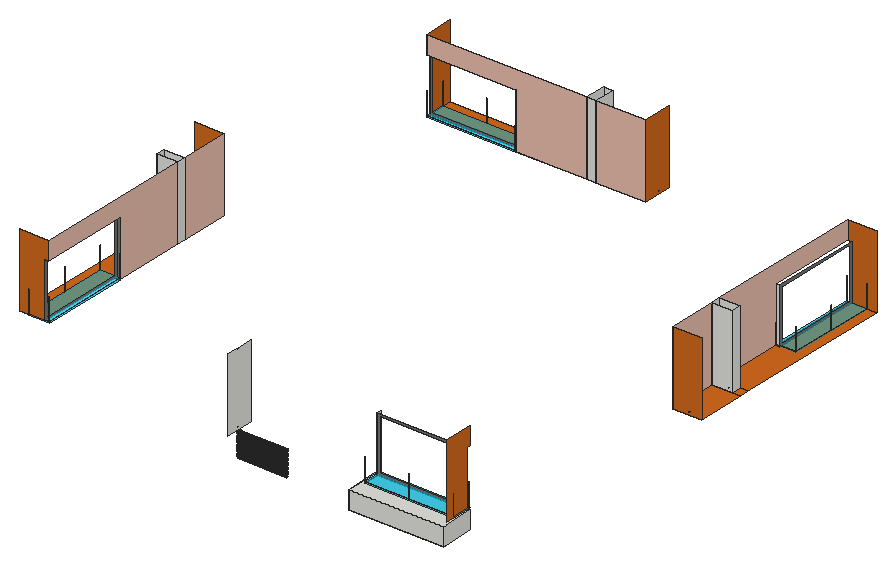
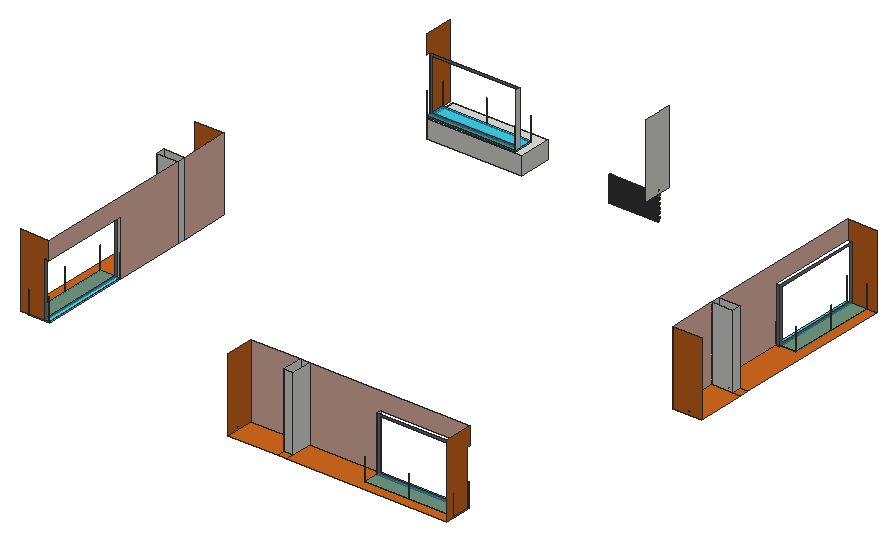
# SketchUp Ruby script. Lengths in inches.
U = 1.inch
M = Sketchup.active_model
def pt(a) = Geom::Point3d.new(a.map { |v| v * U })
def face(e, loops, mat)
  f = e.add_face(loops[0].map { |a| pt(a) })
  loops[1..].each { |l| e.add_face(l.map { |a| pt(a) }).erase! }
  f.material = f.back_material = mat if mat
  f
end
# faces: each face lists its corners as indices into pts; further lists are holes
def faces(e, pts, list, mat = nil) = list.each { |f| face(e, (f[0].is_a?(Array) ? f : [f]).map { |l| l.map { |i| pts[i] } }, mat) }
# xy, xz, yz: faces in a plane at the given z, y or x. An outline is a flat list of corners, or four numbers for a rectangle; further outlines are holes
def ring(l) = l.size == 4 ? [[l[0], l[1]], [l[2], l[1]], [l[2], l[3]], [l[0], l[3]]] : l.each_slice(2).to_a
def flat(e, list, mat, &to3) = list.each { |f| face(e, (f[0].is_a?(Array) ? f : [f]).map { |l| ring(l).map { |u, v| to3.(u, v) } }, mat) }
def xy(e, z, list, mat = nil) = flat(e, list, mat) { |x, y| [x, y, z] }
def xz(e, y, list, mat = nil) = flat(e, list, mat) { |x, z| [x, y, z] }
def yz(e, x, list, mat = nil) = flat(e, list, mat) { |y, z| [x, y, z] }
def lines(e, pts, list) = list.each { |a, b| e.add_line(pt(pts[a]), pt(pts[b])) }
# prism: a flat outline (further loops are holes) pulled along v
def prism(e, loops, v, mat = nil)
  f = face(e, loops, mat); d = Geom::Vector3d.new(v.map { |x| x * U })
  f.pushpull(f.normal.samedirection?(d) ? d.length : -d.length)
end
def box(e, o, s, mat = nil) = prism(e, [[o, [o[0] + s[0], o[1], o[2]], [o[0] + s[0], o[1] + s[1], o[2]], [o[0], o[1] + s[1], o[2]]]], [0, 0, s[2]], mat)
def at(x, y, z, deg = 0) = Geom::Transformation.translation(pt([x, y, z])) * Geom::Transformation.rotation(ORIGIN, Z_AXIS, deg.degrees)
def axes(o, x, y, z) = Geom::Transformation.new([*x, 0, *y, 0, *z, 0, *pt(o).to_a, 1])
def part(name) = M.definitions.add(name)
# library, detail: a bought-in or finely detailed component or shape, given as its bounding box
def library(name, o, s) = part(name).tap { |d| box(d.entities, o, s) }
def detail(e, o, s) = box(e.add_group.entities, o, s)
def put(e, d, t, mat = nil) = e.add_instance(d, t).tap { |i| i.material = mat if mat }
def group(e, t, mat = nil) = e.add_group.tap { |g| g.transformation = t; g.material = mat if mat }.entities
root = M.entities
M.materials.add("[0041_Chocolate]").color = [210, 105, 30]
M.materials.add("[0042_Sienna]").color = [160, 82, 45]
M.materials.add("[0119_RosyBrown]").color = [234, 190, 174]
M.materials.add("[Metal Seamed]").color = [118, 119, 115]
M.materials.add("[Translucent Glass Tinted]").color = [8, 201, 241]
M.materials["[Translucent Glass Tinted]"].alpha = 0.48
c1 = part("Altan")
box(c1.entities,[0,0,0],[118.11,59.06,3.9375])
c2 = part("Staal sojle alta")
box(c2.entities,[0,0,0],[0.87,0.87,43.31])
prism(root,[[[1139,96.8125,1154.11],[1414.89,97.68,1154.11],[1415.2,0.87,1154.11],[1139.3,0,1154.11]]],[0,0,52.19])
xy(root,1213.11,[[72,636.29,132,662.8],[1488,886.83,1548,913.33],[671.48,1452.8125,697.99,1512.8125]])
xy(root,1213.11,[[48,169.92,120,169.92,120,429.61,132,429.61,132,636.29,48,636.29],[48,636.29,72,662.8],[48,662.8,132,806.17],[1488,743.45,1572,886.83],[1548,886.83,1572,913.33],
  [1488,913.33,1572,913.33,1572,1379.7,1500,1379.7,1500,1120.01,1488,1120.01],[464.8,1452.8125,671.48,1452.8125,671.48,1536.8125,205.11,1536.8125,205.11,1464.8125,464.8,1464.8125],[697.99,1452.8125,841.36,1536.8125],[671.48,1512.8125,697.99,1536.8125]],"[0041_Chocolate]")
xy(root,1213.11,[[1155.2,84.8125,1414.89,96.8125]],"[0042_Sienna]")
xz(root,84.8125,[[[1155.2,1213.11,1414.89,1373.61],[1161.2,1219.11,1408.89,1367.61]]],"[Metal Seamed]")
xz(root,169.92,[[48,1213.11,48,1426.89,132,1426.89,132,1373.61,120,1373.61,120,1213.11]],"[0041_Chocolate]")
xz(root,429.61,[[120,1213.11,132,1373.61]],"[Metal Seamed]")
xz(root,636.29,[[72,1213.11,132,1426.89]])
xz(root,662.8,[[[72,1213.11,132,1426.89],[83.53,1218.02,84.48,1218.14,85.37,1218.51,86.13,1219.1,86.72,1219.86,87.09,1220.75,87.21,1221.7,87.09,1222.66,86.72,1223.55,86.13,1224.3125,85.37,1224.9,84.48,1225.27,83.53,1225.39,82.57,1225.27,81.68,1224.9,80.92,1224.3125,80.33,1223.55,79.97,1222.66,79.84,1221.7,79.97,1220.75,80.33,1219.86,80.92,1219.1,81.68,1218.51,82.57,1218.14]]])
xz(root,743.45,[[[1488,1213.11,1572,1426.89],[1536.47,1218.02,1537.43,1218.14,1538.32,1218.51,1539.08,1219.1,1539.67,1219.86,1540.03,1220.75,1540.16,1221.7,1540.03,1222.66,1539.67,1223.55,1539.08,1224.3125,1538.32,1224.9,1537.43,1225.27,1536.47,1225.39,1535.52,1225.27,1534.63,1224.9,1533.87,1224.3125,1533.28,1223.55,1532.91,1222.66,1532.79,1221.7,1532.91,1220.75,1533.28,1219.86,1533.87,1219.1,1534.63,1218.51,1535.52,1218.14]]],"[0041_Chocolate]")
xz(root,806.17,[[[48,1213.11,132,1426.89],[83.53,1218.02,82.57,1218.14,81.68,1218.51,80.92,1219.1,80.33,1219.86,79.97,1220.75,79.84,1221.7,79.97,1222.66,80.33,1223.55,80.92,1224.3125,81.68,1224.9,82.57,1225.27,83.53,1225.39,84.48,1225.27,85.37,1224.9,86.13,1224.3125,86.72,1223.55,87.09,1222.66,87.21,1221.7,87.09,1220.75,86.72,1219.86,86.13,1219.1,85.37,1218.51,84.48,1218.14]]],"[0041_Chocolate]")
xz(root,886.83,[[[1488,1213.11,1548,1426.89],[1536.47,1218.02,1535.52,1218.14,1534.63,1218.51,1533.87,1219.1,1533.28,1219.86,1532.91,1220.75,1532.79,1221.7,1532.91,1222.66,1533.28,1223.55,1533.87,1224.3125,1534.63,1224.9,1535.52,1225.27,1536.47,1225.39,1537.43,1225.27,1538.32,1224.9,1539.08,1224.3125,1539.67,1223.55,1540.03,1222.66,1540.16,1221.7,1540.03,1220.75,1539.67,1219.86,1539.08,1219.1,1538.32,1218.51,1537.43,1218.14]]])
xz(root,913.33,[[1488,1213.11,1548,1426.89]])
xz(root,1120.01,[[1488,1213.11,1500,1373.61]])
xz(root,1379.7,[[1500,1213.11,1572,1213.11,1572,1426.89,1488,1426.89,1488,1373.61,1500,1373.61]],"[0041_Chocolate]")
xz(root,1452.8125,[[671.48,1213.11,697.99,1426.89]])
xz(root,1452.8125,[[464.8,1213.11,464.8,1373.61,205.11,1373.61,205.11,1426.89,671.48,1426.89,671.48,1213.11],[697.99,1213.11,841.36,1426.89]],"[0119_RosyBrown]")
xz(root,1464.8125,[[[205.11,1213.11,464.8,1373.61],[211.11,1219.11,458.8,1367.61]]],"[Metal Seamed]")
xz(root,1512.8125,[[671.48,1213.11,697.99,1426.89]])
yz(root,72,[[636.29,1213.11,662.8,1426.89]])
yz(root,120,[[[169.92,1213.11,429.61,1373.61],[175.92,1219.11,423.61,1367.61]]],"[Metal Seamed]")
yz(root,132,[[636.29,1213.11,662.8,1426.89]])
yz(root,132,[[429.61,1213.11,429.61,1373.61,169.92,1373.61,169.92,1426.89,636.29,1426.89,636.29,1213.11],[662.8,1213.11,806.17,1426.89]],"[0119_RosyBrown]")
yz(root,205.11,[[1464.8125,1213.11,1536.8125,1213.11,1536.8125,1426.89,1452.8125,1426.89,1452.8125,1373.61,1464.8125,1373.61]],"[0041_Chocolate]")
yz(root,464.8,[[1452.8125,1213.11,1464.8125,1373.61]])
yz(root,671.48,[[1452.8125,1213.11,1512.8125,1426.89]])
yz(root,697.99,[[[1452.8125,1213.11,1512.8125,1426.89],[1501.28,1218.02,1500.33,1218.14,1499.44,1218.51,1498.68,1219.1,1498.09,1219.86,1497.72,1220.75,1497.6,1221.7,1497.72,1222.66,1498.09,1223.55,1498.68,1224.3125,1499.44,1224.9,1500.33,1225.27,1501.28,1225.39,1502.24,1225.27,1503.13,1224.9,1503.89,1224.3125,1504.48,1223.55,1504.85,1222.66,1504.97,1221.7,1504.85,1220.75,1504.48,1219.86,1503.89,1219.1,1503.13,1218.51,1502.24,1218.14]]])
yz(root,778.64,[[[12.8125,1213.11,47.01,1213.11,47.38,1213.27,48.34,1213.39,49.29,1213.27,49.67,1213.11,96.8125,1213.11,96.8125,1426.89,51.8,1426.89,51.9,1426.66,52.03,1425.7,51.9,1424.75,51.53,1423.86,50.95,1423.1,50.18,1422.51,49.29,1422.14,48.34,1422.02,47.38,1422.14,46.5,1422.51,45.73,1423.1,45.15,1423.86,44.78,1424.75,44.65,1425.7,44.78,1426.66,44.875,1426.89,12.8125,1426.89],[48.34,1218.02,47.38,1218.14,46.5,1218.51,45.73,1219.1,45.15,1219.86,44.78,1220.75,44.65,1221.7,44.78,1222.66,45.15,1223.55,45.73,1224.3125,46.5,1224.9,47.38,1225.27,48.34,1225.39,49.29,1225.27,50.18,1224.9,50.95,1224.3125,51.53,1223.55,51.9,1222.66,52.03,1221.7,51.9,1220.75,51.53,1219.86,50.95,1219.1,50.18,1218.51,49.29,1218.14]],[47.01,1213.11,49.67,1213.11,49.29,1213.27,48.34,1213.39,47.38,1213.27]])
yz(root,778.64,[[48.34,1206.02,49.29,1206.14,50.18,1206.51,50.95,1207.1,51.53,1207.86,51.9,1208.75,52.03,1209.7,51.9,1210.66,51.53,1211.55,50.95,1212.3125,50.18,1212.9,49.67,1213.11,47.01,1213.11,46.5,1212.9,45.73,1212.3125,45.15,1211.55,44.78,1210.66,44.65,1209.7,44.78,1208.75,45.15,1207.86,45.73,1207.1,46.5,1206.51,47.38,1206.14]],"[0042_Sienna]")
yz(root,841.36,[[[1452.8125,1213.11,1536.8125,1426.89],[1501.28,1218.02,1502.24,1218.14,1503.13,1218.51,1503.89,1219.1,1504.48,1219.86,1504.85,1220.75,1504.97,1221.7,1504.85,1222.66,1504.48,1223.55,1503.89,1224.3125,1503.13,1224.9,1502.24,1225.27,1501.28,1225.39,1500.33,1225.27,1499.44,1224.9,1498.68,1224.3125,1498.09,1223.55,1497.72,1222.66,1497.6,1221.7,1497.72,1220.75,1498.09,1219.86,1498.68,1219.1,1499.44,1218.51,1500.33,1218.14]]],"[0041_Chocolate]")
yz(root,1155.2,[[84.8125,1213.11,96.8125,1373.61]])
yz(root,1414.89,[[12.8125,1213.11,12.8125,1426.89,96.8125,1426.89,96.8125,1373.61,84.8125,1373.61,84.8125,1213.11]],"[0041_Chocolate]")
yz(root,1488,[[886.83,1213.11,913.33,1426.89]])
yz(root,1488,[[743.45,1213.11,886.83,1426.89],[913.33,1213.11,1120.01,1213.11,1120.01,1373.61,1379.7,1373.61,1379.7,1426.89,913.33,1426.89]],"[0119_RosyBrown]")
yz(root,1500,[[[1120.01,1213.11,1379.7,1373.61],[1126.01,1219.11,1373.7,1367.61]]],"[Metal Seamed]")
yz(root,1548,[[886.83,1213.11,913.33,1426.89]])
p = [[922.01,46.5,1140.9],[922.01,47.38,1141.27],[778.64,47.38,1141.27],[778.64,46.5,1140.9],[922.01,49.29,1141.27],[922.01,50.18,1140.9],
  [778.64,50.18,1140.9],[778.64,49.29,1141.27],[922.01,48.34,1141.39],[778.64,48.34,1141.39],[922.01,48.34,1146.02],[922.01,47.38,1146.14],
  [778.64,47.38,1146.14],[778.64,48.34,1146.02],[922.01,49.29,1146.14],[778.64,49.29,1146.14],[922.01,46.5,1146.51],[778.64,46.5,1146.51],
  [922.01,50.18,1146.51],[778.64,50.18,1146.51],[922.01,45.73,1147.1],[778.64,45.73,1147.1],[922.01,50.95,1147.1],[778.64,50.95,1147.1],
  [922.01,45.15,1147.86],[778.64,45.15,1147.86],[922.01,51.53,1147.86],[778.64,51.53,1147.86],[922.01,44.78,1148.75],[778.64,44.78,1148.75],
  [922.01,51.9,1148.75],[778.64,51.9,1148.75],[922.01,44.65,1149.7],[778.64,44.65,1149.7],[922.01,52.03,1149.7],[778.64,52.03,1149.7],
  [922.01,44.78,1150.66],[778.64,44.78,1150.66],[922.01,51.9,1150.66],[778.64,51.9,1150.66],[922.01,45.15,1151.55],[778.64,45.15,1151.55],
  [922.01,51.53,1151.55],[778.64,51.53,1151.55],[922.01,45.73,1152.3125],[778.64,45.73,1152.3125],[922.01,50.95,1152.3125],[778.64,50.95,1152.3125],
  [922.01,46.5,1152.9],[778.64,46.5,1152.9],[922.01,50.18,1152.9],[778.64,50.18,1152.9],[922.01,47.38,1153.27],[778.64,47.38,1153.27],
  [922.01,49.29,1153.27],[778.64,49.29,1153.27],[922.01,48.34,1153.39],[778.64,48.34,1153.39],[922.01,48.34,1158.02],[922.01,47.38,1158.14],
  [778.64,47.38,1158.14],[778.64,48.34,1158.02],[922.01,49.29,1158.14],[778.64,49.29,1158.14],[922.01,46.5,1158.51],[778.64,46.5,1158.51],
  [922.01,50.18,1158.51],[778.64,50.18,1158.51],[922.01,45.73,1159.1],[778.64,45.73,1159.1],[922.01,50.95,1159.1],[778.64,50.95,1159.1],
  [922.01,45.15,1159.86],[778.64,45.15,1159.86],[922.01,51.53,1159.86],[778.64,51.53,1159.86],[922.01,44.78,1160.75],[778.64,44.78,1160.75],
  [922.01,51.9,1160.75],[778.64,51.9,1160.75],[922.01,44.65,1161.7],[778.64,44.65,1161.7],[922.01,52.03,1161.7],[778.64,52.03,1161.7],
  [922.01,44.78,1162.66],[778.64,44.78,1162.66],[922.01,51.9,1162.66],[778.64,51.9,1162.66],[922.01,45.15,1163.55],[778.64,45.15,1163.55],
  [922.01,51.53,1163.55],[778.64,51.53,1163.55],[922.01,45.73,1164.3125],[778.64,45.73,1164.3125],[922.01,50.95,1164.3125],[778.64,50.95,1164.3125],
  [922.01,46.5,1164.9],[778.64,46.5,1164.9],[922.01,50.18,1164.9],[778.64,50.18,1164.9],[922.01,47.38,1165.27],[778.64,47.38,1165.27],
  [922.01,49.29,1165.27],[778.64,49.29,1165.27],[922.01,48.34,1165.39],[778.64,48.34,1165.39],[922.01,48.34,1170.02],[922.01,47.38,1170.14],
  [778.64,47.38,1170.14],[778.64,48.34,1170.02],[922.01,49.29,1170.14],[778.64,49.29,1170.14],[922.01,46.5,1170.51],[778.64,46.5,1170.51],
  [922.01,50.18,1170.51],[778.64,50.18,1170.51],[922.01,45.73,1171.1],[778.64,45.73,1171.1],[922.01,50.95,1171.1],[778.64,50.95,1171.1],
  [922.01,45.15,1171.86],[778.64,45.15,1171.86],[922.01,51.53,1171.86],[778.64,51.53,1171.86],[922.01,44.78,1172.75],[778.64,44.78,1172.75],
  [922.01,51.9,1172.75],[778.64,51.9,1172.75],[922.01,44.65,1173.7],[778.64,44.65,1173.7],[922.01,52.03,1173.7],[778.64,52.03,1173.7],
  [922.01,44.78,1174.66],[778.64,44.78,1174.66],[922.01,51.9,1174.66],[778.64,51.9,1174.66],[922.01,45.15,1175.55],[778.64,45.15,1175.55],
  [922.01,51.53,1175.55],[778.64,51.53,1175.55],[922.01,45.73,1176.3125],[778.64,45.73,1176.3125],[922.01,50.95,1176.3125],[778.64,50.95,1176.3125],
  [922.01,46.5,1176.9],[778.64,46.5,1176.9],[922.01,50.18,1176.9],[778.64,50.18,1176.9],[922.01,47.38,1177.27],[778.64,47.38,1177.27],
  [922.01,49.29,1177.27],[778.64,49.29,1177.27],[922.01,48.34,1177.39],[778.64,48.34,1177.39],[922.01,48.34,1182.02],[922.01,47.38,1182.14],
  [778.64,47.38,1182.14],[778.64,48.34,1182.02],[922.01,49.29,1182.14],[778.64,49.29,1182.14],[922.01,46.5,1182.51],[778.64,46.5,1182.51],
  [922.01,50.18,1182.51],[778.64,50.18,1182.51],[922.01,45.73,1183.1],[778.64,45.73,1183.1],[922.01,50.95,1183.1],[778.64,50.95,1183.1],
  [922.01,45.15,1183.86],[778.64,45.15,1183.86],[922.01,51.53,1183.86],[778.64,51.53,1183.86],[922.01,44.78,1184.75],[778.64,44.78,1184.75],
  [922.01,51.9,1184.75],[778.64,51.9,1184.75],[922.01,44.65,1185.7],[778.64,44.65,1185.7],[922.01,52.03,1185.7],[778.64,52.03,1185.7],
  [922.01,44.78,1186.66],[778.64,44.78,1186.66],[922.01,51.9,1186.66],[778.64,51.9,1186.66],[922.01,45.15,1187.55],[778.64,45.15,1187.55],
  [922.01,51.53,1187.55],[778.64,51.53,1187.55],[922.01,45.73,1188.3125],[778.64,45.73,1188.3125],[922.01,50.95,1188.3125],[778.64,50.95,1188.3125],
  [922.01,46.5,1188.9],[778.64,46.5,1188.9],[922.01,50.18,1188.9],[778.64,50.18,1188.9],[922.01,47.38,1189.27],[778.64,47.38,1189.27],
  [922.01,49.29,1189.27],[778.64,49.29,1189.27],[922.01,48.34,1189.39],[778.64,48.34,1189.39],[922.01,48.34,1194.02],[922.01,47.38,1194.14],
  [778.64,47.38,1194.14],[778.64,48.34,1194.02],[922.01,49.29,1194.14],[778.64,49.29,1194.14],[922.01,46.5,1194.51],[778.64,46.5,1194.51],
  [922.01,50.18,1194.51],[778.64,50.18,1194.51],[922.01,45.73,1195.1],[778.64,45.73,1195.1],[922.01,50.95,1195.1],[778.64,50.95,1195.1],
  [922.01,45.15,1195.86],[778.64,45.15,1195.86],[922.01,51.53,1195.86],[778.64,51.53,1195.86],[922.01,44.78,1196.75],[778.64,44.78,1196.75],
  [922.01,51.9,1196.75],[778.64,51.9,1196.75],[922.01,44.65,1197.7],[778.64,44.65,1197.7],[922.01,52.03,1197.7],[778.64,52.03,1197.7],
  [922.01,44.78,1198.66],[778.64,44.78,1198.66],[922.01,51.9,1198.66],[778.64,51.9,1198.66],[922.01,45.15,1199.55],[778.64,45.15,1199.55],
  [922.01,51.53,1199.55],[778.64,51.53,1199.55],[922.01,45.73,1200.3125],[778.64,45.73,1200.3125],[922.01,50.95,1200.3125],[778.64,50.95,1200.3125],
  [922.01,46.5,1200.9],[778.64,46.5,1200.9],[922.01,50.18,1200.9],[778.64,50.18,1200.9],[922.01,47.38,1201.27],[778.64,47.38,1201.27],
  [922.01,49.29,1201.27],[778.64,49.29,1201.27],[922.01,48.34,1201.39],[778.64,48.34,1201.39],[922.01,48.34,1206.02],[922.01,47.38,1206.14],
  [778.64,47.38,1206.14],[778.64,48.34,1206.02],[922.01,49.29,1206.14],[778.64,49.29,1206.14],[922.01,46.5,1206.51],[778.64,46.5,1206.51],
  [922.01,50.18,1206.51],[778.64,50.18,1206.51],[922.01,45.73,1207.1],[778.64,45.73,1207.1],[922.01,50.95,1207.1],[778.64,50.95,1207.1],
  [922.01,45.15,1207.86],[778.64,45.15,1207.86],[922.01,51.53,1207.86],[778.64,51.53,1207.86],[922.01,44.78,1208.75],[778.64,44.78,1208.75],
  [922.01,51.9,1208.75],[778.64,51.9,1208.75],[922.01,44.65,1209.7],[778.64,44.65,1209.7],[922.01,52.03,1209.7],[778.64,52.03,1209.7],
  [922.01,44.78,1210.66],[778.64,44.78,1210.66],[922.01,51.9,1210.66],[778.64,51.9,1210.66],[922.01,45.15,1211.55],[778.64,45.15,1211.55],
  [922.01,51.53,1211.55],[778.64,51.53,1211.55],[922.01,45.73,1212.3125],[778.64,45.73,1212.3125],[922.01,50.95,1212.3125],[778.64,50.95,1212.3125],
  [922.01,46.5,1212.9],[778.64,46.5,1212.9],[922.01,50.18,1212.9],[778.64,50.18,1212.9],[922.01,47.38,1213.27],[778.64,47.38,1213.27],
  [778.64,47.01,1213.11],[922.01,49.29,1213.27],[778.64,49.67,1213.11],[778.64,49.29,1213.27],[922.01,48.34,1213.39],[778.64,48.34,1213.39]]
faces(root,p,[[0,1,2,3],[4,5,6,7],[1,8,9,2],[8,4,7,9],[10,11,12,13],[14,10,13,15],[11,16,17,12],[18,14,15,19],
  [16,20,21,17],[22,18,19,23],[20,24,25,21],[26,22,23,27],[24,28,29,25],[30,26,27,31],[28,32,33,29],[34,30,31,35],
  [32,36,37,33],[38,34,35,39],[36,40,41,37],[42,38,39,43],[40,44,45,41],[46,42,43,47],[44,48,49,45],[50,46,47,51],
  [48,52,53,49],[54,50,51,55],[52,56,57,53],[56,54,55,57],[58,59,60,61],[62,58,61,63],[59,64,65,60],[66,62,63,67],
  [64,68,69,65],[70,66,67,71],[68,72,73,69],[74,70,71,75],[72,76,77,73],[78,74,75,79],[76,80,81,77],[82,78,79,83],
  [80,84,85,81],[86,82,83,87],[84,88,89,85],[90,86,87,91],[88,92,93,89],[94,90,91,95],[92,96,97,93],[98,94,95,99],
  [96,100,101,97],[102,98,99,103],[100,104,105,101],[104,102,103,105],[106,107,108,109],[110,106,109,111],[107,112,113,108],[114,110,111,115],
  [112,116,117,113],[118,114,115,119],[116,120,121,117],[122,118,119,123],[120,124,125,121],[126,122,123,127],[124,128,129,125],[130,126,127,131],
  [128,132,133,129],[134,130,131,135],[132,136,137,133],[138,134,135,139],[136,140,141,137],[142,138,139,143],[140,144,145,141],[146,142,143,147],
  [144,148,149,145],[150,146,147,151],[148,152,153,149],[152,150,151,153],[154,155,156,157],[158,154,157,159],[155,160,161,156],[162,158,159,163],
  [160,164,165,161],[166,162,163,167],[164,168,169,165],[170,166,167,171],[168,172,173,169],[174,170,171,175],[172,176,177,173],[178,174,175,179],
  [176,180,181,177],[182,178,179,183],[180,184,185,181],[186,182,183,187],[184,188,189,185],[190,186,187,191],[188,192,193,189],[194,190,191,195],
  [192,196,197,193],[198,194,195,199],[196,200,201,197],[200,198,199,201],[202,203,204,205],[206,202,205,207],[203,208,209,204],[210,206,207,211],
  [208,212,213,209],[214,210,211,215],[212,216,217,213],[218,214,215,219],[216,220,221,217],[222,218,219,223],[220,224,225,221],[226,222,223,227],
  [224,228,229,225],[230,226,227,231],[228,232,233,229],[234,230,231,235],[232,236,237,233],[238,234,235,239],[236,240,241,237],[242,238,239,243],
  [240,244,245,241],[246,242,243,247],[244,248,249,245],[248,246,247,249],[250,251,252,253],[254,250,253,255],[251,256,257,252],[258,254,255,259],
  [256,260,261,257],[262,258,259,263],[260,264,265,261],[266,262,263,267],[264,268,269,265],[270,266,267,271],[268,272,273,269],[274,270,271,275],
  [272,276,277,273],[278,274,275,279],[276,280,281,277],[282,278,279,283],[280,284,285,281],[286,282,283,287],[284,288,289,285],[290,286,287,291],
  [288,292,293,294,289],[295,290,291,296,297],[292,298,299,293],[298,295,297,299]])
put(root,c1,axes([1487.13,1379.7,1209.17],[0,-2.19843,0],[1,0,0],[0,0,1.5]),"[Translucent Glass Tinted]")
put(root,c1,axes([1414.89,97.68,1209.17],[-2.19843,0,0],[0,-1,0],[0,0,1.5]),"[Translucent Glass Tinted]")
put(root,c1,axes([132.87,169.92,1209.17],[0,2.19843,0],[-1,0,0],[0,0,1.5]),"[Translucent Glass Tinted]")
put(root,c1,axes([205.11,1451.94,1209.17],[2.19843,0,0],[0,1,0],[0,0,1.5]),"[Translucent Glass Tinted]")
put(root,c2,axes([132.87,427.66,1215.08],[0,2.19843,0],[-1,0,0],[0,0,1.5]),"[Translucent Glass Tinted]")
put(root,c2,axes([205.11,1510.125,1215.08],[2.19843,0,0],[0,1,0],[0,0,1.5]),"[Translucent Glass Tinted]")
put(root,c2,axes([1286.12,39.5,1215.08],[-2.19843,0,0],[0,-1,0],[0,0,1.5]),"[Translucent Glass Tinted]")
put(root,c2,axes([74.69,169.92,1215.08],[0,2.19843,0],[-1,0,0],[0,0,1.5]),"[Translucent Glass Tinted]")
put(root,c2,axes([1545.31,1121.96,1215.08],[0,-2.19843,0],[1,0,0],[0,0,1.5]),"[Translucent Glass Tinted]")
put(root,c2,axes([1545.31,1250.93,1215.08],[0,-2.19843,0],[1,0,0],[0,0,1.5]),"[Translucent Glass Tinted]")
put(root,c2,axes([1545.31,1379.7,1215.08],[0,-2.19843,0],[1,0,0],[0,0,1.5]),"[Translucent Glass Tinted]")
put(root,c2,axes([1414.89,97.68,1215.08],[-2.19843,0,0],[0,-1,0],[0,0,1.5]),"[Translucent Glass Tinted]")
put(root,c2,axes([74.69,298.69,1215.08],[0,2.19843,0],[-1,0,0],[0,0,1.5]),"[Translucent Glass Tinted]")
put(root,c2,axes([74.69,427.66,1215.08],[0,2.19843,0],[-1,0,0],[0,0,1.5]),"[Translucent Glass Tinted]")
put(root,c2,axes([1414.89,39.5,1215.08],[-2.19843,0,0],[0,-1,0],[0,0,1.5]),"[Translucent Glass Tinted]")
put(root,c2,axes([333.88,1510.125,1215.08],[2.19843,0,0],[0,1,0],[0,0,1.5]),"[Translucent Glass Tinted]")
put(root,c2,axes([1487.13,1121.96,1215.08],[0,-2.19843,0],[1,0,0],[0,0,1.5]),"[Translucent Glass Tinted]")
put(root,c2,axes([462.85,1451.94,1215.08],[2.19843,0,0],[0,1,0],[0,0,1.5]),"[Translucent Glass Tinted]")
put(root,c2,axes([1157.15,39.5,1215.08],[-2.19843,0,0],[0,-1,0],[0,0,1.5]),"[Translucent Glass Tinted]")
put(root,c2,axes([462.85,1510.125,1215.08],[2.19843,0,0],[0,1,0],[0,0,1.5]),"[Translucent Glass Tinted]")
put(root,c2,axes([1487.13,1379.7,1215.08],[0,-2.19843,0],[1,0,0],[0,0,1.5]),"[Translucent Glass Tinted]")
put(root,c2,axes([132.87,169.92,1215.08],[0,2.19843,0],[-1,0,0],[0,0,1.5]),"[Translucent Glass Tinted]")
put(root,c2,axes([205.11,1451.94,1215.08],[2.19843,0,0],[0,1,0],[0,0,1.5]),"[Translucent Glass Tinted]")
put(root,c2,axes([1157.15,97.68,1215.08],[-2.19843,0,0],[0,-1,0],[0,0,1.5]),"[Translucent Glass Tinted]")
